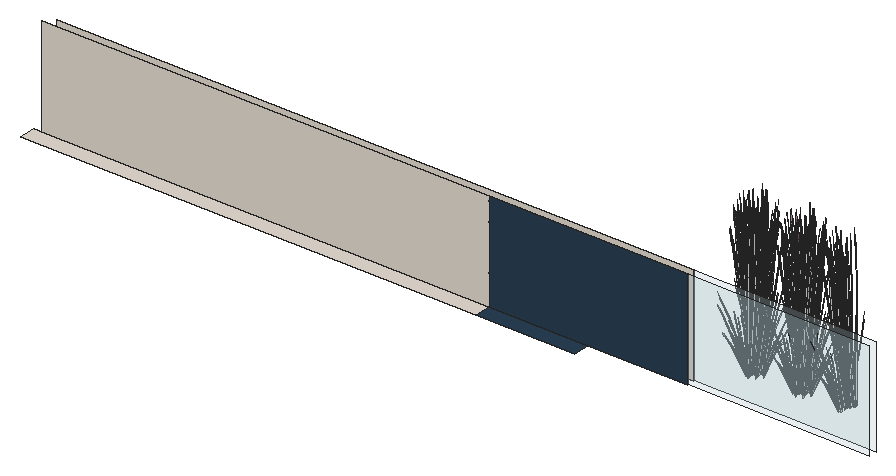
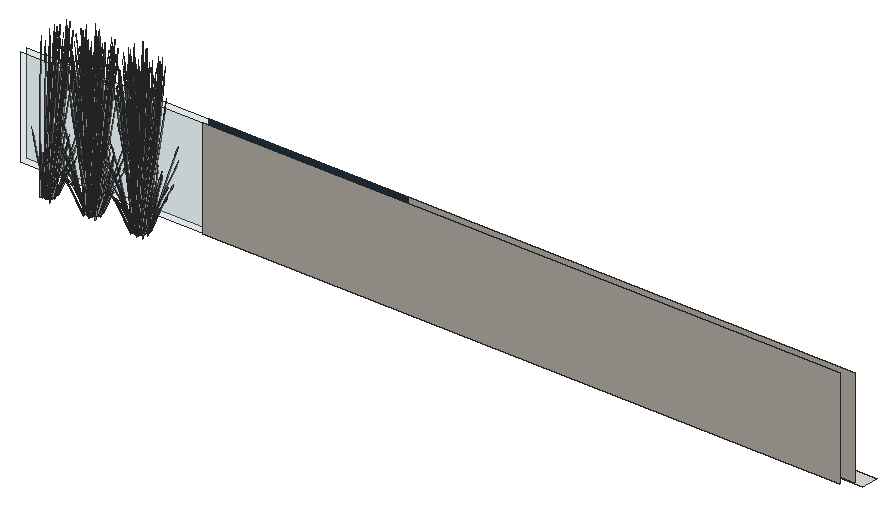
# SketchUp Ruby script. Lengths in inches.
U = 1.inch
M = Sketchup.active_model
def pt(a) = Geom::Point3d.new(a.map { |v| v * U })
def face(e, loops, mat)
  f = e.add_face(loops[0].map { |a| pt(a) })
  loops[1..].each { |l| e.add_face(l.map { |a| pt(a) }).erase! }
  f.material = f.back_material = mat if mat
  f
end
# faces: each face lists its corners as indices into pts; further lists are holes
def faces(e, pts, list, mat = nil) = list.each { |f| face(e, (f[0].is_a?(Array) ? f : [f]).map { |l| l.map { |i| pts[i] } }, mat) }
# xy, xz, yz: faces in a plane at the given z, y or x. An outline is a flat list of corners, or four numbers for a rectangle; further outlines are holes
def ring(l) = l.size == 4 ? [[l[0], l[1]], [l[2], l[1]], [l[2], l[3]], [l[0], l[3]]] : l.each_slice(2).to_a
def flat(e, list, mat, &to3) = list.each { |f| face(e, (f[0].is_a?(Array) ? f : [f]).map { |l| ring(l).map { |u, v| to3.(u, v) } }, mat) }
def xy(e, z, list, mat = nil) = flat(e, list, mat) { |x, y| [x, y, z] }
def xz(e, y, list, mat = nil) = flat(e, list, mat) { |x, z| [x, y, z] }
def yz(e, x, list, mat = nil) = flat(e, list, mat) { |y, z| [x, y, z] }
def lines(e, pts, list) = list.each { |a, b| e.add_line(pt(pts[a]), pt(pts[b])) }
# prism: a flat outline (further loops are holes) pulled along v
def prism(e, loops, v, mat = nil)
  f = face(e, loops, mat); d = Geom::Vector3d.new(v.map { |x| x * U })
  f.pushpull(f.normal.samedirection?(d) ? d.length : -d.length)
end
def box(e, o, s, mat = nil) = prism(e, [[o, [o[0] + s[0], o[1], o[2]], [o[0] + s[0], o[1] + s[1], o[2]], [o[0], o[1] + s[1], o[2]]]], [0, 0, s[2]], mat)
def at(x, y, z, deg = 0) = Geom::Transformation.translation(pt([x, y, z])) * Geom::Transformation.rotation(ORIGIN, Z_AXIS, deg.degrees)
def axes(o, x, y, z) = Geom::Transformation.new([*x, 0, *y, 0, *z, 0, *pt(o).to_a, 1])
def part(name) = M.definitions.add(name)
# library, detail: a bought-in or finely detailed component or shape, given as its bounding box
def library(name, o, s) = part(name).tap { |d| box(d.entities, o, s) }
def detail(e, o, s) = box(e.add_group.entities, o, s)
def put(e, d, t, mat = nil) = e.add_instance(d, t).tap { |i| i.material = mat if mat }
def group(e, t, mat = nil) = e.add_group.tap { |g| g.transformation = t; g.material = mat if mat }.entities
root = M.entities
M.materials.add("Carpet_04_1K").color = [43, 65, 85]
M.materials.add("Glass_Safety_01").color = [204, 235, 244]
M.materials["Glass_Safety_01"].alpha = 0.25
M.materials.add("LightPink_Translucent").color = [144, 107, 117]
M.materials["LightPink_Translucent"].alpha = 0.75
M.materials.add("Marble_01_1K").color = [230, 221, 211]
c1 = part("blade")
p = [[2.15,0.21,22],[0,0.17,0],[0.09,0.45,0],[2.18,0.31,22],[2.29,0.31,22],[0.38,0.45,0],
  [2.48,0.24,33],[2.49,0.24,33],[2.48,0.22,33]]
faces(c1.entities,p,[[0,1,2,3],[4,5,2,3],[6,3,4,7],[8,0,3,6]])
c2 = part("seeds")
p = [[0.3,-0.1,1.38],[-0.01,-0.03,1.59],[-0.01,-0.03,0.03],[0.14,-0.07,-0.07],[0.29,-0.03,3],[0.15,0.01,3.11]]
faces(c2.entities,p,[[0,1,2,3],[1,0,4,5]],"LightPink_Translucent")
c3 = part("blade with seeds")
put(c3.entities,c1,at(0,0,0))
put(c3.entities,c2,axes([2.4,0.25,30.99],[1.5799,-0.05474,1.17369],[-0.12525,1.92788,0.29478],[-0.07173,-0.02425,1.56792]))
xy(root,264,[[201,36,237,42]],"Carpet_04_1K")
xy(root,264,[[36,36,201,42]],"Marble_01_1K")
xz(root,42,[[201,264,273,300]],"Carpet_04_1K")
xz(root,42,[[273,264,339,300]],"Glass_Safety_01")
xz(root,42,[[39,264,201,300]],"Marble_01_1K")
xz(root,45,[[273,264,338.95,300]],"Glass_Safety_01")
xz(root,45,[[42,264,273,300]],"Marble_01_1K")
put(root,c3,axes([282.76,58.17,266.41],[0.17773,0.04462,1.33163],[0.11455,0.45576,-0.28638],[-0.24142,0.08531,0.56934]))
put(root,c3,axes([283.45,55.97,266.41],[0.09985,0.15133,1.33163],[-0.23008,0.41134,-0.28638],[-0.23625,-0.09832,0.56934]))
put(root,c3,axes([283.09,56.98,265.39],[0.01297,0.08566,1.6421],[-0.26146,0.44735,-0.25086],[-0.18572,-0.02255,0.2797]))
put(root,c3,axes([282.39,59.125,266.58],[0.21313,-0.24635,1.06958],[0.0841,0.38999,0.78586],[-0.15402,0.06983,0.23558]))
put(root,c3,axes([282.95,59.38,265.39],[0.0686,0.0543,1.6421],[0.11632,0.50315,-0.25086],[-0.15204,0.10729,0.2797]))
put(root,c3,axes([282.86,56.42,266.58],[0.3265,-0.03889,1.06958],[-0.20711,0.3427,0.78586],[-0.16135,-0.05141,0.23558]))
put(root,c3,axes([284.8,57.76,265.92],[-0.53199,-0.08911,-0.58063],[0.11226,-0.54969,-0.15239],[-0.15876,-0.06661,1.28164]))
put(root,c3,axes([284.11,58.8,265.88],[-0.47863,-0.27177,-0.46235],[0.28609,-0.48733,0],[-0.10901,-0.0619,1.46668]))
put(root,c3,axes([283.9,54.75,265.39],[-0.04954,0.0716,1.6421],[-0.50062,0.15438,-0.25086],[-0.12094,-0.14044,0.2797]))
put(root,c3,axes([284.4,59.125,266.21],[-0.31974,0.54466,0],[-0.53494,-0.30375,-0.48057],[-0.12184,-0.06918,1.52448]))
put(root,c3,axes([283.8125,59.91,266.41],[0.16138,-0.08575,1.33163],[0.39845,0.25854,-0.28638],[-0.1186,0.22371,0.56934]))
put(root,c3,axes([283.58,55.03,265.98],[-0.14753,0.44383,-0.03625],[-0.45406,-0.13653,-0.16435],[-0.06894,-0.07259,0.54209]))
put(root,c3,axes([284.26,54.47,266.41],[-0.03097,0.17781,1.33163],[-0.45273,0.14885,-0.28638],[-0.10583,-0.22982,0.56934]))
put(root,c3,axes([285.41,57.84,266.48],[-0.51635,0.36087,-0.27094],[-0.34336,-0.5099,-0.46562],[-0.1274,-0.05178,1.4872]))
put(root,c3,axes([283.34,57.05,266.21],[-0.63949,0,0],[0,-0.60749,-0.48057],[0,-0.13836,1.52448]))
put(root,c3,axes([284.24,58.59,265.89],[-0.12013,-0.47362,-0.28847],[0.47712,-0.13449,0.28847],[-0.09619,-0.05462,1.29413]))
put(root,c3,axes([285.75,58.23,265.92],[-0.34446,0.40855,-0.58063],[-0.42791,-0.37046,-0.15239],[-0.13803,0.10191,1.28164]))
put(root,c3,axes([283.84,56.89,266.17],[-0.47569,0.45698,0.2864],[-0.47598,-0.45217,-0.33981],[-0.01661,-0.12977,1.53541]))
put(root,c3,axes([284.11,54.18,266.58],[0.26677,0.18918,1.06958],[-0.38851,0.11372,0.78586],[-0.08313,-0.14539,0.23558]))
put(root,c3,axes([285.99,58,266.3],[-0.49938,-0.43748,-0.23459],[0.42021,-0.49126,0.51337],[-0.13447,0.05118,1.56642]))
put(root,c3,axes([285.08,57.58,266.06],[-0.30722,-0.45622,-0.41661],[0.46535,-0.32126,0.2005],[-0.09942,-0.05645,1.33761]))
put(root,c3,axes([284.2,60.2,266.58],[-0.01324,-0.32319,1.06958],[0.33072,0.23052,0.78586],[-0.06504,0.15405,0.23558]))
put(root,c3,axes([285.73,57.91,266.06],[-0.55535,0.03355,-0.41661],[-0.05022,-0.55698,0.2005],[-0.09942,0.05645,1.33761]))
put(root,c3,axes([284.67,58.84,266.31],[0.47863,0.27177,0.46235],[-0.28609,0.48733,0],[-0.10901,-0.0619,1.46668]))
put(root,c3,axes([285.125,57.84,266.27],[0.13555,-0.64407,-0.21817],[0.64269,0.11227,0.47743],[-0.1123,-0.08895,1.45677]))
put(root,c3,axes([285.36,58,266.4375],[-0.09866,0.48509,0.13483],[-0.48202,-0.0842,-0.38503],[-0.08772,-0.04981,1.18024]))
put(root,c3,axes([286.32,59.35,265.88],[-0.47863,0.27177,-0.46235],[-0.28609,-0.48733,0],[-0.10901,0.0619,1.46668]))
put(root,c3,axes([283.48,56.64,265.88],[0,-0.54355,-0.46235],[0.57217,0,0],[0,-0.1238,1.46668]))
put(root,c3,axes([283.73,57.14,266.31],[0,0.54355,0.46235],[-0.57217,0,0],[0,-0.1238,1.46668]))
put(root,c3,axes([286.35,59.2,266.04],[-0.31576,-0.54657,-0.04789],[0.53494,-0.30375,0.48057],[-0.13182,0.05204,1.52373]))
put(root,c3,axes([286.2,59.13,265.89],[-0.47712,-0.13449,-0.28847],[0.12013,-0.47362,0.28847],[-0.09619,0.05462,1.29413]))
put(root,c3,axes([284.98,57.27,266.48],[-0.57594,-0.25935,-0.27094],[0.27732,-0.5474,-0.46562],[-0.0181,-0.1344,1.4872]))
put(root,c3,axes([283.93,59.5,266.63],[0.46459,-0.09625,0.0606],[0.10681,0.38778,-0.80367],[-0.02945,0.1963,0.72038]))
put(root,c3,axes([286.125,57.76,266.48],[0.05959,0.62022,-0.27094],[-0.62068,0.0375,-0.46562],[-0.1093,0.08261,1.4872]))
put(root,c3,axes([284.72,56.72,265.95],[-0.21003,-0.55738,-0.65031],[0.60499,-0.20074,-0.17068],[-0.02321,-0.18874,1.43544]))
put(root,c3,axes([283.73,56.65,265.89],[0.35699,-0.33913,-0.28847],[0.35699,0.33913,0.28847],[0,-0.10923,1.29413]))
put(root,c3,axes([285.34,54.46,265.98],[-0.35341,0.31182,-0.03625],[-0.32382,-0.34152,-0.16435],[-0.0228,-0.09677,0.54209]))
put(root,c3,axes([285.2,57.53,266.2],[0.64638,0.11452,0.42607],[-0.13155,0.64678,0.16719],[-0.09446,-0.06245,1.47927]))
put(root,c3,axes([285.03,57.42,266.53],[-0.24813,0.48978,0.41661],[-0.51557,-0.23571,-0.2005],[0,-0.1129,1.33761]))
put(root,c3,axes([284.85,58.57,266.3],[0.54955,-0.14427,0.16428],[0.1357,0.53689,0.32672],[-0.04901,-0.07823,1.49371]))
put(root,c3,axes([285.56,58.65,266.05],[-0.51557,-0.24403,0],[0.24813,-0.50705,0],[0,0,1.51513]))
put(root,c3,axes([286.75,59.26,266.21],[0.31974,0.54466,0],[-0.53494,0.30375,-0.48057],[-0.12184,0.06918,1.52448]))
put(root,c3,axes([286.49,58.6,266.3],[0.14774,-0.54019,0.16428],[0.54062,0.15287,0.32672],[-0.09339,0.00263,1.49371]))
put(root,c3,axes([286.24,57.88,266.4375],[0.37783,0.32657,0.13483],[-0.31516,0.36844,-0.38503],[-0.08772,0.04981,1.18024]))
put(root,c3,axes([286.1,57.48,266.14],[-0.47569,-0.46784,-0.05709],[0.47598,-0.46812,0],[-0.01661,-0.01634,1.63492]))
put(root,c3,axes([286.23,57.64,266.53],[0.55535,-0.03355,0.41661],[0.05022,0.55698,-0.2005],[-0.09942,0.05645,1.33761]))
put(root,c3,axes([286.36,58.92,266.17],[0.64025,0.17667,0.2864],[-0.16018,0.63149,-0.33981],[-0.10597,0.07904,1.53541]))
put(root,c3,axes([285.43,54.08,265.39],[-0.08578,0.01958,1.6421],[-0.47437,-0.22044,-0.25086],[0.00796,-0.18387,0.2797]))
put(root,c3,axes([286.64,58.89,266.31],[0.47863,-0.27177,0.46235],[0.28609,0.48733,0],[-0.10901,0.0619,1.46668]))
put(root,c3,axes([285.14,56.9375,266.2],[0.22235,0.6078,0.42607],[-0.63531,0.21135,0.16719],[0.00776,-0.11168,1.47927]))
put(root,c3,axes([285.04,56.86,266.06],[0.24813,-0.48978,-0.41661],[0.51557,0.23571,0.2005],[0,-0.1129,1.33761]))
put(root,c3,axes([285.68,58.44,266.05],[-0.16686,-0.46861,0],[0.47648,-0.16411,0],[0,0,1.4375]))
put(root,c3,axes([285.07,59.43,265.39],[0.08277,-0.02958,1.6421],[0.49786,0.16279,-0.25086],[0.01456,0.18348,0.2797]))
put(root,c3,axes([286.35,57.52,266.06],[-0.24813,0.48978,-0.41661],[-0.51557,-0.23571,0.2005],[0,0.1129,1.33761]))
put(root,c3,axes([287.33,57.22,266.3],[-0.40181,-0.39593,0.16428],[0.40492,-0.38402,0.32672],[-0.04438,0.08086,1.49371]))
put(root,c3,axes([285.94,56.99,266.05],[0,-0.62892,0],[0.63949,0,0],[0,0,1.6711]))
put(root,c3,axes([285.35,57.1,266.27],[0.57623,0.26344,0.22409],[-0.27732,0.5474,0.46562],[0,-0.12618,1.49497]))
put(root,c3,axes([286.26,57.24,266.13],[0,0.62861,-0.05249],[-0.63949,0,0],[0,0.01975,1.67027]))
put(root,c3,axes([285.16,56.74,266.53],[-0.55535,0.03355,0.41661],[-0.05022,-0.55698,-0.2005],[0.09942,-0.05645,1.33761]))
put(root,c3,axes([284.9,55.78,266.3],[-0.14774,0.54019,0.16428],[-0.54062,-0.15287,0.32672],[0.09339,-0.00263,1.49371]))
put(root,c3,axes([285.96,58.46,266.13],[0.22235,0.62444,-0.05599],[-0.63531,0.21881,0],[0.00776,0.02181,1.60327]))
put(root,c3,axes([284.64,55.11,266.21],[-0.31974,-0.54466,0],[0.53494,-0.30375,-0.48057],[0.12184,-0.06918,1.52448]))
put(root,c3,axes([287.79,57.64,266.05],[-0.63917,-0.00435,-0.04634],[0,-0.60749,0.46507],[-0.02009,0.13829,1.47457]))
put(root,c3,axes([286.54,55.8125,266.3],[-0.54955,0.14427,0.16428],[-0.1357,-0.53689,0.32672],[0.04901,0.07823,1.49371]))
put(root,c3,axes([285.98,53.8,266.58],[0.06561,0.31695,1.06958],[-0.36394,-0.17555,0.78586],[0.03916,-0.16229,0.23558]))
put(root,c3,axes([285.64,56.59,266.2],[-0.42403,0.49328,0.42607],[-0.50377,-0.43543,0.16719],[0.10223,-0.04923,1.47927]))
put(root,c3,axes([286.36,57.37,266.0625],[0.35699,0.35109,0],[-0.35699,0.35109,0],[0,0,1.57621]))
put(root,c3,axes([286.36,56.96,266.53],[0.24813,-0.48978,0.41661],[0.51557,0.23571,-0.2005],[0,0.1129,1.33761]))
put(root,c3,axes([286.14,58.66,266.05],[0.51557,0.24403,0],[-0.24813,0.50705,0],[0,0,1.62917]))
put(root,c3,axes([286.19,56.84,266.22],[-0.64638,-0.11452,0.45814],[0.13155,-0.64678,0.17978],[0.09446,0.06245,1.59061]))
put(root,c3,axes([287.66,57.73,265.89],[-0.35699,0.33913,-0.28847],[-0.35699,-0.33913,0.28847],[0,0.10923,1.29413]))
put(root,c3,axes([286.64,57.66,265.95],[0.18752,0.49766,-0.6445],[-0.54017,0.17923,-0.16915],[0.02073,0.16852,1.42262]))
put(root,c3,axes([286.375,57.13,266.05],[0.57217,0,0],[0,0.56272,0],[0,0,1.66132]))
put(root,c3,axes([285.83,56.51,266.53],[-0.30722,-0.45622,0.41661],[0.46535,-0.32126,-0.2005],[0.09942,0.05645,1.33761]))
put(root,c3,axes([285.27,56.62,266.48],[-0.05959,-0.62022,-0.27094],[0.62068,-0.0375,-0.46562],[0.1093,-0.08261,1.4872]))
put(root,c3,axes([286.57,57.07,266.4375],[0.47648,-0.15851,0.13483],[0.16686,0.45265,-0.38503],[0,0.09962,1.18024]))
put(root,c3,axes([286.41,57.11,266.48],[0.57594,0.25935,-0.27094],[-0.27732,0.5474,-0.46562],[0.0181,0.1344,1.4872]))
put(root,c3,axes([285.19,55.25,265.89],[0.47712,0.13449,-0.28847],[-0.12013,0.47362,0.28847],[0.09619,-0.05462,1.29413]))
put(root,c3,axes([286.51,54.67,266.41],[-0.14537,0.11002,1.33163],[-0.43536,-0.19256,-0.28638],[0.0807,-0.23948,0.56934]))
put(root,c3,axes([287.66,57.23,266.31],[0,-0.54355,0.46235],[0.57217,0,0],[0,0.1238,1.46668]))
put(root,c3,axes([287.91,57.74,265.88],[0,0.54355,-0.46235],[-0.57217,0,0],[0,0.1238,1.46668]))
put(root,c3,axes([285.07,55.03,265.88],[0.47863,-0.27177,-0.46235],[0.28609,0.48733,0],[0.10901,-0.0619,1.46668]))
put(root,c3,axes([286.03,56.38,266.4375],[0.09866,-0.48509,0.13483],[0.48202,0.0842,-0.38503],[0.08772,0.04981,1.18024]))
put(root,c3,axes([286.72,55.54,266.31],[-0.47863,-0.27177,0.46235],[0.28609,-0.48733,0],[0.10901,0.0619,1.46668]))
put(root,c3,axes([286.3,58.375,266.03],[0.53691,-0.18442,-0.17877],[0.18866,0.53125,0.00007],[0.05927,-0.02038,1.61933]))
put(root,c3,axes([286.3125,56.8,266.06],[0.30722,0.45622,-0.41661],[-0.46535,0.32126,0.2005],[0.09942,0.05645,1.33761]))
put(root,c3,axes([287.18,58.87,266.58],[-0.28795,-0.15629,1.06958],[0.37181,-0.1588,0.78586],[0.10029,0.13452,0.23558]))
put(root,c3,axes([286.16,58.7,266.41],[0.00902,-0.18018,1.33163],[0.43127,-0.20126,-0.28638],[0.13313,0.21566,0.56934]))
put(root,c3,axes([285.64,56.15,265.92],[0.34446,-0.40855,-0.58063],[0.42791,0.37046,-0.15239],[0.13803,-0.10191,1.28164]))
put(root,c3,axes([287.15,55.78,265.89],[0.12013,0.47362,-0.28847],[-0.47712,0.13449,0.28847],[0.09619,0.05462,1.29413]))
put(root,c3,axes([288.05,57.33,266.21],[0.63949,0,0],[0,0.60749,-0.48057],[0,0.13836,1.52448]))
put(root,c3,axes([285.98,56.54,266.48],[0.51635,-0.36087,-0.27094],[0.34336,0.5099,-0.46562],[0.1274,0.05178,1.4872]))
put(root,c3,axes([287.23,59.58,266.48],[-0.32795,-0.01705,0.97832],[0.21658,-0.36206,0.54015],[0.12956,0.12863,0.76741]))
put(root,c3,axes([284.68,56.22,265.48],[-0.50338,0.21762,1.20058],[-0.16022,-0.62439,0.4665],[0.30911,0.01039,1.36553]))
put(root,c3,axes([286.99,55.25,266.21],[0.31974,-0.54466,0],[0.53494,0.30375,-0.48057],[0.12184,0.06918,1.52448]))
put(root,c3,axes([287.53,55.01,265.39],[-0.07655,-0.04282,1.6421],[-0.19662,-0.47839,-0.25086],[0.13264,-0.12982,0.2797]))
put(root,c3,axes([287.28,55.58,265.88],[0.47863,0.27177,-0.46235],[-0.28609,0.48733,0],[0.10901,0.0619,1.46668]))
put(root,c3,axes([287.26,59.45,265.39],[0.03726,-0.07847,1.6421],[0.46909,-0.23111,-0.25086],[0.14221,0.11962,0.2797]))
put(root,c3,axes([286.59,56.62,265.92],[0.53199,0.08911,-0.58063],[-0.11226,0.54969,-0.15239],[0.15876,0.06661,1.28164]))
put(root,c3,axes([288.85,56.94,266.11],[-0.31706,-0.34757,-0.06041],[0.34725,-0.31847,-0.27392],[0.09839,-0.02242,0.90349]))
put(root,c3,axes([288.125,55.18,266.58],[-0.17034,0.27669,1.06958],[-0.14642,-0.37174,0.78586],[0.14069,-0.09315,0.23558]))
put(root,c3,axes([288.9375,57.58,266.58],[-0.31598,0.08973,1.06958],[0.14873,-0.37085,0.78586],[0.16763,0.02538,0.23558]))
put(root,c3,axes([287.91,55.97,266.41],[-0.1827,-0.0161,1.33163],[-0.18717,-0.43188,-0.28638],[0.22444,-0.12218,0.56934]))
put(root,c3,axes([288.25,57.4,265.85],[-0.32938,0.06523,1.31842],[-0.05243,-0.51922,0.07547],[0.2307,-0.07859,0.75023]))
put(root,c3,axes([288.61,57.07,265.39],[-0.02673,-0.08252,1.6421],[0.18538,-0.48271,-0.25086],[0.187,-0.00694,0.2797]))
put(root,c3,axes([288.34,58.18,266.41],[-0.12317,-0.13368,1.33163],[0.16025,-0.44223,-0.28638],[0.24919,0.05991,0.56934]))
put(root,c3,axes([299.98,58.17,266.41],[0.17773,0.04462,1.33163],[0.11455,0.45576,-0.28638],[-0.24142,0.08531,0.56934]))
put(root,c3,axes([300.67,55.97,266.41],[0.09985,0.15133,1.33163],[-0.23008,0.41134,-0.28638],[-0.23625,-0.09832,0.56934]))
put(root,c3,axes([300.3125,56.98,265.39],[0.01297,0.08566,1.6421],[-0.26146,0.44735,-0.25086],[-0.18572,-0.02255,0.2797]))
put(root,c3,axes([299.61,59.125,266.58],[0.21313,-0.24635,1.06958],[0.0841,0.38999,0.78586],[-0.15402,0.06983,0.23558]))
put(root,c3,axes([300.17,59.38,265.39],[0.0686,0.0543,1.6421],[0.11632,0.50315,-0.25086],[-0.15204,0.10729,0.2797]))
put(root,c3,axes([300.07,56.42,266.58],[0.3265,-0.03889,1.06958],[-0.20711,0.3427,0.78586],[-0.16135,-0.05141,0.23558]))
put(root,c3,axes([302.02,57.76,265.92],[-0.53199,-0.08911,-0.58063],[0.11226,-0.54969,-0.15239],[-0.15876,-0.06661,1.28164]))
put(root,c3,axes([301.32,58.8,265.88],[-0.47863,-0.27177,-0.46235],[0.28609,-0.48733,0],[-0.10901,-0.0619,1.46668]))
put(root,c3,axes([301.11,54.75,265.39],[-0.04954,0.0716,1.6421],[-0.50062,0.15438,-0.25086],[-0.12094,-0.14044,0.2797]))
put(root,c3,axes([301.62,59.125,266.21],[-0.31974,0.54466,0],[-0.53494,-0.30375,-0.48057],[-0.12184,-0.06918,1.52448]))
put(root,c3,axes([301.03,59.91,266.41],[0.16138,-0.08575,1.33163],[0.39845,0.25854,-0.28638],[-0.1186,0.22371,0.56934]))
put(root,c3,axes([300.8,55.03,265.98],[-0.14753,0.44383,-0.03625],[-0.45406,-0.13653,-0.16435],[-0.06894,-0.07259,0.54209]))
put(root,c3,axes([301.48,54.47,266.41],[-0.03097,0.17781,1.33163],[-0.45273,0.14885,-0.28638],[-0.10583,-0.22982,0.56934]))
put(root,c3,axes([302.625,57.84,266.48],[-0.51635,0.36087,-0.27094],[-0.34336,-0.5099,-0.46562],[-0.1274,-0.05178,1.4872]))
put(root,c3,axes([300.56,57.05,266.21],[-0.63949,0,0],[0,-0.60749,-0.48057],[0,-0.13836,1.52448]))
put(root,c3,axes([301.46,58.59,265.89],[-0.12013,-0.47362,-0.28847],[0.47712,-0.13449,0.28847],[-0.09619,-0.05462,1.29413]))
put(root,c3,axes([302.97,58.23,265.92],[-0.34446,0.40855,-0.58063],[-0.42791,-0.37046,-0.15239],[-0.13803,0.10191,1.28164]))
put(root,c3,axes([301.06,56.89,266.17],[-0.47569,0.45698,0.2864],[-0.47598,-0.45217,-0.33981],[-0.01661,-0.12977,1.53541]))
put(root,c3,axes([301.33,54.18,266.58],[0.26677,0.18918,1.06958],[-0.38851,0.11372,0.78586],[-0.08313,-0.14539,0.23558]))
put(root,c3,axes([303.21,58,266.3],[-0.49938,-0.43748,-0.23459],[0.42021,-0.49126,0.51337],[-0.13447,0.05118,1.56642]))
put(root,c3,axes([302.3,57.58,266.06],[-0.30722,-0.45622,-0.41661],[0.46535,-0.32126,0.2005],[-0.09942,-0.05645,1.33761]))
put(root,c3,axes([301.42,60.2,266.58],[-0.01324,-0.32319,1.06958],[0.33072,0.23052,0.78586],[-0.06504,0.15405,0.23558]))
put(root,c3,axes([302.95,57.91,266.06],[-0.55535,0.03355,-0.41661],[-0.05022,-0.55698,0.2005],[-0.09942,0.05645,1.33761]))
put(root,c3,axes([301.89,58.84,266.31],[0.47863,0.27177,0.46235],[-0.28609,0.48733,0],[-0.10901,-0.0619,1.46668]))
put(root,c3,axes([302.34,57.84,266.27],[0.13555,-0.64407,-0.21817],[0.64269,0.11227,0.47743],[-0.1123,-0.08895,1.45677]))
put(root,c3,axes([302.58,58,266.4375],[-0.09866,0.48509,0.13483],[-0.48202,-0.0842,-0.38503],[-0.08772,-0.04981,1.18024]))
put(root,c3,axes([303.54,59.35,265.88],[-0.47863,0.27177,-0.46235],[-0.28609,-0.48733,0],[-0.10901,0.0619,1.46668]))
put(root,c3,axes([300.7,56.64,265.88],[0,-0.54355,-0.46235],[0.57217,0,0],[0,-0.1238,1.46668]))
put(root,c3,axes([300.95,57.14,266.31],[0,0.54355,0.46235],[-0.57217,0,0],[0,-0.1238,1.46668]))
put(root,c3,axes([303.57,59.2,266.04],[-0.31576,-0.54657,-0.04789],[0.53494,-0.30375,0.48057],[-0.13182,0.05204,1.52373]))
put(root,c3,axes([303.42,59.13,265.89],[-0.47712,-0.13449,-0.28847],[0.12013,-0.47362,0.28847],[-0.09619,0.05462,1.29413]))
put(root,c3,axes([302.2,57.27,266.48],[-0.57594,-0.25935,-0.27094],[0.27732,-0.5474,-0.46562],[-0.0181,-0.1344,1.4872]))
put(root,c3,axes([301.15,59.5,266.63],[0.46459,-0.09625,0.0606],[0.10681,0.38778,-0.80367],[-0.02945,0.1963,0.72038]))
put(root,c3,axes([303.34,57.76,266.48],[0.05959,0.62022,-0.27094],[-0.62068,0.0375,-0.46562],[-0.1093,0.08261,1.4872]))
put(root,c3,axes([301.94,56.72,265.95],[-0.21003,-0.55738,-0.65031],[0.60499,-0.20074,-0.17068],[-0.02321,-0.18874,1.43544]))
put(root,c3,axes([300.95,56.65,265.89],[0.35699,-0.33913,-0.28847],[0.35699,0.33913,0.28847],[0,-0.10923,1.29413]))
put(root,c3,axes([302.56,54.46,265.98],[-0.35341,0.31182,-0.03625],[-0.32382,-0.34152,-0.16435],[-0.0228,-0.09677,0.54209]))
put(root,c3,axes([302.42,57.53,266.2],[0.64638,0.11452,0.42607],[-0.13155,0.64678,0.16719],[-0.09446,-0.06245,1.47927]))
put(root,c3,axes([302.25,57.42,266.53],[-0.24813,0.48978,0.41661],[-0.51557,-0.23571,-0.2005],[0,-0.1129,1.33761]))
put(root,c3,axes([302.07,58.57,266.3],[0.54955,-0.14427,0.16428],[0.1357,0.53689,0.32672],[-0.04901,-0.07823,1.49371]))
put(root,c3,axes([302.78,58.65,266.05],[-0.51557,-0.24403,0],[0.24813,-0.50705,0],[0,0,1.51513]))
put(root,c3,axes([303.97,59.26,266.21],[0.31974,0.54466,0],[-0.53494,0.30375,-0.48057],[-0.12184,0.06918,1.52448]))
put(root,c3,axes([303.71,58.6,266.3],[0.14774,-0.54019,0.16428],[0.54062,0.15287,0.32672],[-0.09339,0.00263,1.49371]))
put(root,c3,axes([303.46,57.88,266.4375],[0.37783,0.32657,0.13483],[-0.31516,0.36844,-0.38503],[-0.08772,0.04981,1.18024]))
put(root,c3,axes([303.32,57.48,266.14],[-0.47569,-0.46784,-0.05709],[0.47598,-0.46812,0],[-0.01661,-0.01634,1.63492]))
put(root,c3,axes([303.45,57.64,266.53],[0.55535,-0.03355,0.41661],[0.05022,0.55698,-0.2005],[-0.09942,0.05645,1.33761]))
put(root,c3,axes([303.58,58.92,266.17],[0.64025,0.17667,0.2864],[-0.16018,0.63149,-0.33981],[-0.10597,0.07904,1.53541]))
put(root,c3,axes([302.65,54.08,265.39],[-0.08578,0.01958,1.6421],[-0.47437,-0.22044,-0.25086],[0.00796,-0.18387,0.2797]))
put(root,c3,axes([303.86,58.89,266.31],[0.47863,-0.27177,0.46235],[0.28609,0.48733,0],[-0.10901,0.0619,1.46668]))
put(root,c3,axes([302.36,56.9375,266.2],[0.22235,0.6078,0.42607],[-0.63531,0.21135,0.16719],[0.00776,-0.11168,1.47927]))
put(root,c3,axes([302.26,56.86,266.06],[0.24813,-0.48978,-0.41661],[0.51557,0.23571,0.2005],[0,-0.1129,1.33761]))
put(root,c3,axes([302.9,58.44,266.05],[-0.16686,-0.46861,0],[0.47648,-0.16411,0],[0,0,1.4375]))
put(root,c3,axes([302.29,59.43,265.39],[0.08277,-0.02958,1.6421],[0.49786,0.16279,-0.25086],[0.01456,0.18348,0.2797]))
put(root,c3,axes([303.57,57.52,266.06],[-0.24813,0.48978,-0.41661],[-0.51557,-0.23571,0.2005],[0,0.1129,1.33761]))
put(root,c3,axes([304.55,57.22,266.3],[-0.40181,-0.39593,0.16428],[0.40492,-0.38402,0.32672],[-0.04438,0.08086,1.49371]))
put(root,c3,axes([303.16,56.99,266.05],[0,-0.62892,0],[0.63949,0,0],[0,0,1.6711]))
put(root,c3,axes([302.57,57.1,266.27],[0.57623,0.26344,0.22409],[-0.27732,0.5474,0.46562],[0,-0.12618,1.49497]))
put(root,c3,axes([303.48,57.24,266.13],[0,0.62861,-0.05249],[-0.63949,0,0],[0,0.01975,1.67027]))
put(root,c3,axes([302.38,56.74,266.53],[-0.55535,0.03355,0.41661],[-0.05022,-0.55698,-0.2005],[0.09942,-0.05645,1.33761]))
put(root,c3,axes([302.12,55.78,266.3],[-0.14774,0.54019,0.16428],[-0.54062,-0.15287,0.32672],[0.09339,-0.00263,1.49371]))
put(root,c3,axes([303.18,58.46,266.13],[0.22235,0.62444,-0.05599],[-0.63531,0.21881,0],[0.00776,0.02181,1.60327]))
put(root,c3,axes([301.86,55.11,266.21],[-0.31974,-0.54466,0],[0.53494,-0.30375,-0.48057],[0.12184,-0.06918,1.52448]))
put(root,c3,axes([305.01,57.64,266.05],[-0.63917,-0.00435,-0.04634],[0,-0.60749,0.46507],[-0.02009,0.13829,1.47457]))
put(root,c3,axes([303.76,55.8125,266.3],[-0.54955,0.14427,0.16428],[-0.1357,-0.53689,0.32672],[0.04901,0.07823,1.49371]))
put(root,c3,axes([303.2,53.8,266.58],[0.06561,0.31695,1.06958],[-0.36394,-0.17555,0.78586],[0.03916,-0.16229,0.23558]))
put(root,c3,axes([302.86,56.59,266.2],[-0.42403,0.49328,0.42607],[-0.50377,-0.43543,0.16719],[0.10223,-0.04923,1.47927]))
put(root,c3,axes([303.58,57.37,266.0625],[0.35699,0.35109,0],[-0.35699,0.35109,0],[0,0,1.57621]))
put(root,c3,axes([303.58,56.96,266.53],[0.24813,-0.48978,0.41661],[0.51557,0.23571,-0.2005],[0,0.1129,1.33761]))
put(root,c3,axes([303.36,58.66,266.05],[0.51557,0.24403,0],[-0.24813,0.50705,0],[0,0,1.62917]))
put(root,c3,axes([303.41,56.84,266.22],[-0.64638,-0.11452,0.45814],[0.13155,-0.64678,0.17978],[0.09446,0.06245,1.59061]))
put(root,c3,axes([304.88,57.73,265.89],[-0.35699,0.33913,-0.28847],[-0.35699,-0.33913,0.28847],[0,0.10923,1.29413]))
put(root,c3,axes([303.86,57.66,265.95],[0.18752,0.49766,-0.6445],[-0.54017,0.17923,-0.16915],[0.02073,0.16852,1.42262]))
put(root,c3,axes([303.6,57.13,266.05],[0.57217,0,0],[0,0.56272,0],[0,0,1.66132]))
put(root,c3,axes([303.05,56.51,266.53],[-0.30722,-0.45622,0.41661],[0.46535,-0.32126,-0.2005],[0.09942,0.05645,1.33761]))
put(root,c3,axes([302.49,56.62,266.48],[-0.05959,-0.62022,-0.27094],[0.62068,-0.0375,-0.46562],[0.1093,-0.08261,1.4872]))
put(root,c3,axes([303.79,57.07,266.4375],[0.47648,-0.15851,0.13483],[0.16686,0.45265,-0.38503],[0,0.09962,1.18024]))
put(root,c3,axes([303.63,57.11,266.48],[0.57594,0.25935,-0.27094],[-0.27732,0.5474,-0.46562],[0.0181,0.1344,1.4872]))
put(root,c3,axes([302.4,55.25,265.89],[0.47712,0.13449,-0.28847],[-0.12013,0.47362,0.28847],[0.09619,-0.05462,1.29413]))
put(root,c3,axes([303.73,54.67,266.41],[-0.14537,0.11002,1.33163],[-0.43536,-0.19256,-0.28638],[0.0807,-0.23948,0.56934]))
put(root,c3,axes([304.88,57.23,266.31],[0,-0.54355,0.46235],[0.57217,0,0],[0,0.1238,1.46668]))
put(root,c3,axes([305.125,57.74,265.88],[0,0.54355,-0.46235],[-0.57217,0,0],[0,0.1238,1.46668]))
put(root,c3,axes([302.29,55.03,265.88],[0.47863,-0.27177,-0.46235],[0.28609,0.48733,0],[0.10901,-0.0619,1.46668]))
put(root,c3,axes([303.25,56.38,266.4375],[0.09866,-0.48509,0.13483],[0.48202,0.0842,-0.38503],[0.08772,0.04981,1.18024]))
put(root,c3,axes([303.9375,55.54,266.31],[-0.47863,-0.27177,0.46235],[0.28609,-0.48733,0],[0.10901,0.0619,1.46668]))
put(root,c3,axes([303.52,58.375,266.03],[0.53691,-0.18442,-0.17877],[0.18866,0.53125,0.00007],[0.05927,-0.02038,1.61933]))
put(root,c3,axes([303.53,56.8,266.06],[0.30722,0.45622,-0.41661],[-0.46535,0.32126,0.2005],[0.09942,0.05645,1.33761]))
put(root,c3,axes([304.4,58.87,266.58],[-0.28795,-0.15629,1.06958],[0.37181,-0.1588,0.78586],[0.10029,0.13452,0.23558]))
put(root,c3,axes([303.375,58.7,266.41],[0.00902,-0.18018,1.33163],[0.43127,-0.20126,-0.28638],[0.13313,0.21566,0.56934]))
put(root,c3,axes([302.86,56.15,265.92],[0.34446,-0.40855,-0.58063],[0.42791,0.37046,-0.15239],[0.13803,-0.10191,1.28164]))
put(root,c3,axes([304.37,55.78,265.89],[0.12013,0.47362,-0.28847],[-0.47712,0.13449,0.28847],[0.09619,0.05462,1.29413]))
put(root,c3,axes([305.27,57.33,266.21],[0.63949,0,0],[0,0.60749,-0.48057],[0,0.13836,1.52448]))
put(root,c3,axes([303.2,56.54,266.48],[0.51635,-0.36087,-0.27094],[0.34336,0.5099,-0.46562],[0.1274,0.05178,1.4872]))
put(root,c3,axes([304.45,59.58,266.48],[-0.32795,-0.01705,0.97832],[0.21658,-0.36206,0.54015],[0.12956,0.12863,0.76741]))
put(root,c3,axes([301.9,56.22,265.48],[-0.50338,0.21762,1.20058],[-0.16022,-0.62439,0.4665],[0.30911,0.01039,1.36553]))
put(root,c3,axes([304.21,55.25,266.21],[0.31974,-0.54466,0],[0.53494,0.30375,-0.48057],[0.12184,0.06918,1.52448]))
put(root,c3,axes([304.75,55.01,265.39],[-0.07655,-0.04282,1.6421],[-0.19662,-0.47839,-0.25086],[0.13264,-0.12982,0.2797]))
put(root,c3,axes([304.5,55.58,265.88],[0.47863,0.27177,-0.46235],[-0.28609,0.48733,0],[0.10901,0.0619,1.46668]))
put(root,c3,axes([304.48,59.45,265.39],[0.03726,-0.07847,1.6421],[0.46909,-0.23111,-0.25086],[0.14221,0.11962,0.2797]))
put(root,c3,axes([303.81,56.62,265.92],[0.53199,0.08911,-0.58063],[-0.11226,0.54969,-0.15239],[0.15876,0.06661,1.28164]))
put(root,c3,axes([306.07,56.94,266.11],[-0.31706,-0.34757,-0.06041],[0.34725,-0.31847,-0.27392],[0.09839,-0.02242,0.90349]))
put(root,c3,axes([305.34,55.18,266.58],[-0.17034,0.27669,1.06958],[-0.14642,-0.37174,0.78586],[0.14069,-0.09315,0.23558]))
put(root,c3,axes([306.16,57.58,266.58],[-0.31598,0.08973,1.06958],[0.14873,-0.37085,0.78586],[0.16763,0.02538,0.23558]))
put(root,c3,axes([305.13,55.97,266.41],[-0.1827,-0.0161,1.33163],[-0.18717,-0.43188,-0.28638],[0.22444,-0.12218,0.56934]))
put(root,c3,axes([305.47,57.4,265.85],[-0.32938,0.06523,1.31842],[-0.05243,-0.51922,0.07547],[0.2307,-0.07859,0.75023]))
put(root,c3,axes([305.83,57.07,265.39],[-0.02673,-0.08252,1.6421],[0.18538,-0.48271,-0.25086],[0.187,-0.00694,0.2797]))
put(root,c3,axes([305.56,58.18,266.41],[-0.12317,-0.13368,1.33163],[0.16025,-0.44223,-0.28638],[0.24919,0.05991,0.56934]))
put(root,c3,axes([316.35,58.17,266.41],[0.17773,0.04462,1.33163],[0.11455,0.45576,-0.28638],[-0.24142,0.08531,0.56934]))
put(root,c3,axes([317.03,55.97,266.41],[0.09985,0.15133,1.33163],[-0.23008,0.41134,-0.28638],[-0.23625,-0.09832,0.56934]))
put(root,c3,axes([316.68,56.98,265.39],[0.01297,0.08566,1.6421],[-0.26146,0.44735,-0.25086],[-0.18572,-0.02255,0.2797]))
put(root,c3,axes([315.97,59.125,266.58],[0.21313,-0.24635,1.06958],[0.0841,0.38999,0.78586],[-0.15402,0.06983,0.23558]))
put(root,c3,axes([316.54,59.38,265.39],[0.0686,0.0543,1.6421],[0.11632,0.50315,-0.25086],[-0.15204,0.10729,0.2797]))
put(root,c3,axes([316.4375,56.42,266.58],[0.3265,-0.03889,1.06958],[-0.20711,0.3427,0.78586],[-0.16135,-0.05141,0.23558]))
put(root,c3,axes([318.39,57.76,265.92],[-0.53199,-0.08911,-0.58063],[0.11226,-0.54969,-0.15239],[-0.15876,-0.06661,1.28164]))
put(root,c3,axes([317.6875,58.8,265.88],[-0.47863,-0.27177,-0.46235],[0.28609,-0.48733,0],[-0.10901,-0.0619,1.46668]))
put(root,c3,axes([317.48,54.75,265.39],[-0.04954,0.0716,1.6421],[-0.50062,0.15438,-0.25086],[-0.12094,-0.14044,0.2797]))
put(root,c3,axes([317.98,59.125,266.21],[-0.31974,0.54466,0],[-0.53494,-0.30375,-0.48057],[-0.12184,-0.06918,1.52448]))
put(root,c3,axes([317.4,59.91,266.41],[0.16138,-0.08575,1.33163],[0.39845,0.25854,-0.28638],[-0.1186,0.22371,0.56934]))
put(root,c3,axes([317.17,55.03,265.98],[-0.14753,0.44383,-0.03625],[-0.45406,-0.13653,-0.16435],[-0.06894,-0.07259,0.54209]))
put(root,c3,axes([317.85,54.47,266.41],[-0.03097,0.17781,1.33163],[-0.45273,0.14885,-0.28638],[-0.10583,-0.22982,0.56934]))
put(root,c3,axes([318.99,57.84,266.48],[-0.51635,0.36087,-0.27094],[-0.34336,-0.5099,-0.46562],[-0.1274,-0.05178,1.4872]))
put(root,c3,axes([316.92,57.05,266.21],[-0.63949,0,0],[0,-0.60749,-0.48057],[0,-0.13836,1.52448]))
put(root,c3,axes([317.82,58.59,265.89],[-0.12013,-0.47362,-0.28847],[0.47712,-0.13449,0.28847],[-0.09619,-0.05462,1.29413]))
put(root,c3,axes([319.33,58.23,265.92],[-0.34446,0.40855,-0.58063],[-0.42791,-0.37046,-0.15239],[-0.13803,0.10191,1.28164]))
put(root,c3,axes([317.42,56.89,266.17],[-0.47569,0.45698,0.2864],[-0.47598,-0.45217,-0.33981],[-0.01661,-0.12977,1.53541]))
put(root,c3,axes([317.6875,54.18,266.58],[0.26677,0.18918,1.06958],[-0.38851,0.11372,0.78586],[-0.08313,-0.14539,0.23558]))
put(root,c3,axes([319.57,58,266.3],[-0.49938,-0.43748,-0.23459],[0.42021,-0.49126,0.51337],[-0.13447,0.05118,1.56642]))
put(root,c3,axes([318.66,57.58,266.06],[-0.30722,-0.45622,-0.41661],[0.46535,-0.32126,0.2005],[-0.09942,-0.05645,1.33761]))
put(root,c3,axes([317.78,60.2,266.58],[-0.01324,-0.32319,1.06958],[0.33072,0.23052,0.78586],[-0.06504,0.15405,0.23558]))
put(root,c3,axes([319.32,57.91,266.06],[-0.55535,0.03355,-0.41661],[-0.05022,-0.55698,0.2005],[-0.09942,0.05645,1.33761]))
put(root,c3,axes([318.26,58.84,266.31],[0.47863,0.27177,0.46235],[-0.28609,0.48733,0],[-0.10901,-0.0619,1.46668]))
put(root,c3,axes([318.71,57.84,266.27],[0.13555,-0.64407,-0.21817],[0.64269,0.11227,0.47743],[-0.1123,-0.08895,1.45677]))
put(root,c3,axes([318.94,58,266.4375],[-0.09866,0.48509,0.13483],[-0.48202,-0.0842,-0.38503],[-0.08772,-0.04981,1.18024]))
put(root,c3,axes([319.9,59.35,265.88],[-0.47863,0.27177,-0.46235],[-0.28609,-0.48733,0],[-0.10901,0.0619,1.46668]))
put(root,c3,axes([317.07,56.64,265.88],[0,-0.54355,-0.46235],[0.57217,0,0],[0,-0.1238,1.46668]))
put(root,c3,axes([317.3125,57.14,266.31],[0,0.54355,0.46235],[-0.57217,0,0],[0,-0.1238,1.46668]))
put(root,c3,axes([319.93,59.2,266.04],[-0.31576,-0.54657,-0.04789],[0.53494,-0.30375,0.48057],[-0.13182,0.05204,1.52373]))
put(root,c3,axes([319.79,59.13,265.89],[-0.47712,-0.13449,-0.28847],[0.12013,-0.47362,0.28847],[-0.09619,0.05462,1.29413]))
put(root,c3,axes([318.5625,57.27,266.48],[-0.57594,-0.25935,-0.27094],[0.27732,-0.5474,-0.46562],[-0.0181,-0.1344,1.4872]))
put(root,c3,axes([317.51,59.5,266.63],[0.46459,-0.09625,0.0606],[0.10681,0.38778,-0.80367],[-0.02945,0.1963,0.72038]))
put(root,c3,axes([319.71,57.76,266.48],[0.05959,0.62022,-0.27094],[-0.62068,0.0375,-0.46562],[-0.1093,0.08261,1.4872]))
put(root,c3,axes([318.3,56.72,265.95],[-0.21003,-0.55738,-0.65031],[0.60499,-0.20074,-0.17068],[-0.02321,-0.18874,1.43544]))
put(root,c3,axes([317.3125,56.65,265.89],[0.35699,-0.33913,-0.28847],[0.35699,0.33913,0.28847],[0,-0.10923,1.29413]))
put(root,c3,axes([318.92,54.46,265.98],[-0.35341,0.31182,-0.03625],[-0.32382,-0.34152,-0.16435],[-0.0228,-0.09677,0.54209]))
put(root,c3,axes([318.78,57.53,266.2],[0.64638,0.11452,0.42607],[-0.13155,0.64678,0.16719],[-0.09446,-0.06245,1.47927]))
put(root,c3,axes([318.61,57.42,266.53],[-0.24813,0.48978,0.41661],[-0.51557,-0.23571,-0.2005],[0,-0.1129,1.33761]))
put(root,c3,axes([318.43,58.57,266.3],[0.54955,-0.14427,0.16428],[0.1357,0.53689,0.32672],[-0.04901,-0.07823,1.49371]))
put(root,c3,axes([319.14,58.65,266.05],[-0.51557,-0.24403,0],[0.24813,-0.50705,0],[0,0,1.51513]))
put(root,c3,axes([320.33,59.26,266.21],[0.31974,0.54466,0],[-0.53494,0.30375,-0.48057],[-0.12184,0.06918,1.52448]))
